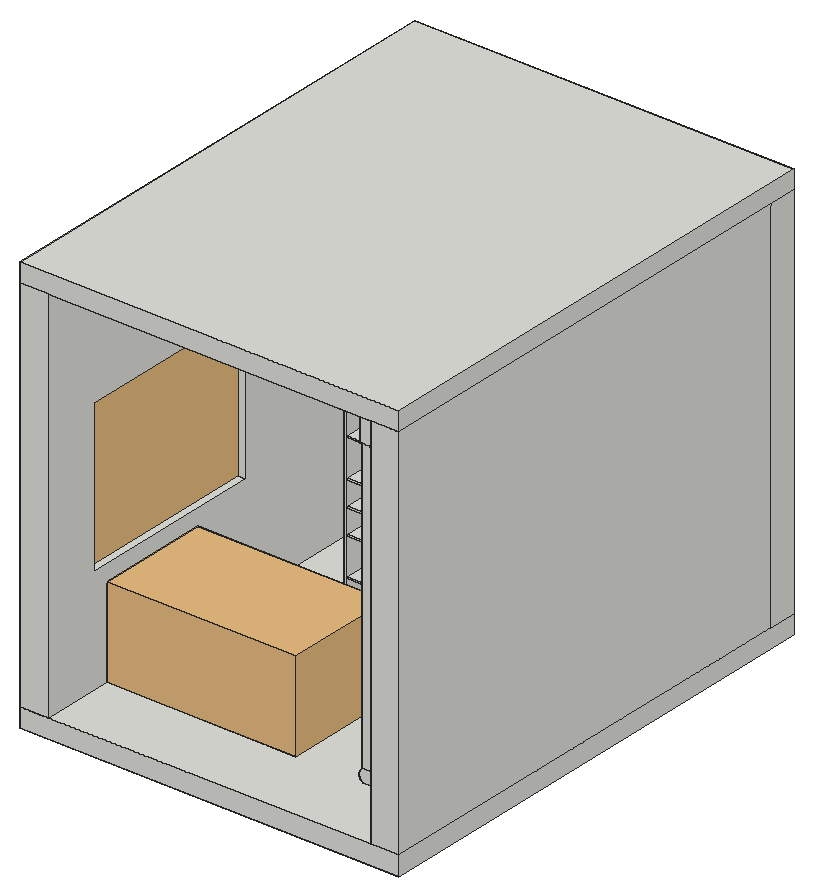
# SketchUp Ruby script. Lengths in inches.
U = 1.inch
M = Sketchup.active_model
def pt(a) = Geom::Point3d.new(a.map { |v| v * U })
def face(e, loops, mat)
  f = e.add_face(loops[0].map { |a| pt(a) })
  loops[1..].each { |l| e.add_face(l.map { |a| pt(a) }).erase! }
  f.material = f.back_material = mat if mat
  f
end
# faces: each face lists its corners as indices into pts; further lists are holes
def faces(e, pts, list, mat = nil) = list.each { |f| face(e, (f[0].is_a?(Array) ? f : [f]).map { |l| l.map { |i| pts[i] } }, mat) }
# xy, xz, yz: faces in a plane at the given z, y or x. An outline is a flat list of corners, or four numbers for a rectangle; further outlines are holes
def ring(l) = l.size == 4 ? [[l[0], l[1]], [l[2], l[1]], [l[2], l[3]], [l[0], l[3]]] : l.each_slice(2).to_a
def flat(e, list, mat, &to3) = list.each { |f| face(e, (f[0].is_a?(Array) ? f : [f]).map { |l| ring(l).map { |u, v| to3.(u, v) } }, mat) }
def xy(e, z, list, mat = nil) = flat(e, list, mat) { |x, y| [x, y, z] }
def xz(e, y, list, mat = nil) = flat(e, list, mat) { |x, z| [x, y, z] }
def yz(e, x, list, mat = nil) = flat(e, list, mat) { |y, z| [x, y, z] }
def lines(e, pts, list) = list.each { |a, b| e.add_line(pt(pts[a]), pt(pts[b])) }
# prism: a flat outline (further loops are holes) pulled along v
def prism(e, loops, v, mat = nil)
  f = face(e, loops, mat); d = Geom::Vector3d.new(v.map { |x| x * U })
  f.pushpull(f.normal.samedirection?(d) ? d.length : -d.length)
end
def box(e, o, s, mat = nil) = prism(e, [[o, [o[0] + s[0], o[1], o[2]], [o[0] + s[0], o[1] + s[1], o[2]], [o[0], o[1] + s[1], o[2]]]], [0, 0, s[2]], mat)
def at(x, y, z, deg = 0) = Geom::Transformation.translation(pt([x, y, z])) * Geom::Transformation.rotation(ORIGIN, Z_AXIS, deg.degrees)
def axes(o, x, y, z) = Geom::Transformation.new([*x, 0, *y, 0, *z, 0, *pt(o).to_a, 1])
def part(name) = M.definitions.add(name)
# library, detail: a bought-in or finely detailed component or shape, given as its bounding box
def library(name, o, s) = part(name).tap { |d| box(d.entities, o, s) }
def detail(e, o, s) = box(e.add_group.entities, o, s)
def put(e, d, t, mat = nil) = e.add_instance(d, t).tap { |i| i.material = mat if mat }
def group(e, t, mat = nil) = e.add_group.tap { |g| g.transformation = t; g.material = mat if mat }.entities
root = M.entities
M.materials.add("[Color C01]").color = [255, 229, 204]
c1 = library("36\" LINEAR DRAIN",[0,0,0],[36,3.67,1.375])
c2 = library("vaso sanitario",[83.83,-83.27,-7.09],[14.69,23.62,31.37])
c3 = library("Health Faucet",[-0.24,4.77,0],[3.42,7.46,21.65])
c4 = library("CUA SO 1",[-70.87,1.66,4.22],[70.87,3.46,66.92])
c5 = library("Casaco",[0,0,0],[25.87,38.71,37.25])
c6 = part("Group\#13")
box(c6.entities,[0,0,0],[9,19,0.5])
c7 = part("Group\#15")
box(c7.entities,[0,0,0],[21,46.71,0.5])
c8 = library("Grupuj\#4",[0,0.09,0],[19.96,5.84,7.875])
c9 = library("Grupuj\#16",[0,0,0],[1.8,5.91,8.5])
c10 = library("Różnica",[0,0,0],[1.2,1.2,6.8])
c11 = part("Grupuj\#13")
xz(c11.entities,0,[[0.78,0.08,0.96,0.1,1.125,0.17,1.27,0.28,1.38,0.43,1.45,0.6,1.48,0.78,1.45,0.96,1.38,1.125,1.27,1.27,1.125,1.38,0.96,1.45,0.78,1.48,0.6,1.45,0.43,1.38,0.28,1.27,0.17,1.125,0.1,0.96,0.08,0.78,0.1,0.6,0.17,0.43,0.28,0.28,0.43,0.17,0.6,0.1]])
xz(c11.entities,1.22,[[0.78,0,0.58,0.03,0.39,0.1,0.23,0.23,0.1,0.39,0.03,0.58,0,0.78,0.03,0.98,0.1,1.17,0.23,1.33,0.39,1.45,0.58,1.53,0.78,1.56,0.98,1.53,1.17,1.45,1.33,1.33,1.45,1.17,1.53,0.98,1.56,0.78,1.53,0.58,1.45,0.39,1.33,0.23,1.17,0.1,0.98,0.03]])
p = [[0.6,0,0.1],[0.43,0,0.17],[0.39,0.08,0.1],[0.58,0.08,0.03],[0.78,0,0.08],[0.78,0.08,0],
  [0.96,0,0.1],[0.98,0.08,0.03],[1.125,0,0.17],[1.17,0.08,0.1],[0.58,1.22,0.03],[0.39,1.22,0.1],
  [0.78,1.22,0],[0.98,1.22,0.03],[1.17,1.22,0.1],[0.28,0,0.28],[0.23,0.08,0.23],[1.27,0,0.28],
  [1.33,0.08,0.23],[0.23,1.22,0.23],[1.33,1.22,0.23],[0.17,0,0.43],[0.1,0.08,0.39],[1.38,0,0.43],
  [1.45,0.08,0.39],[0.1,1.22,0.39],[1.45,1.22,0.39],[0.1,0,0.6],[0.03,0.08,0.58],[1.45,0,0.6],
  [1.53,0.08,0.58],[0.03,1.22,0.58],[1.53,1.22,0.58],[0.08,0,0.78],[0,0.08,0.78],[1.48,0,0.78],
  [1.56,0.08,0.78],[0,1.22,0.78],[1.56,1.22,0.78],[0.1,0,0.96],[0.03,0.08,0.98],[1.45,0,0.96],
  [1.53,0.08,0.98],[0.03,1.22,0.98],[1.53,1.22,0.98],[0.17,0,1.125],[0.1,0.08,1.17],[1.38,0,1.125],
  [1.45,0.08,1.17],[0.1,1.22,1.17],[1.45,1.22,1.17],[0.28,0,1.27],[0.23,0.08,1.33],[1.27,0,1.27],
  [1.33,0.08,1.33],[0.23,1.22,1.33],[1.33,1.22,1.33],[0.43,0,1.38],[0.39,0.08,1.45],[1.125,0,1.38],
  [1.17,0.08,1.45],[0.39,1.22,1.45],[1.17,1.22,1.45],[0.6,0,1.45],[0.58,0.08,1.53],[0.96,0,1.45],
  [0.98,0.08,1.53],[0.78,0,1.48],[0.78,0.08,1.56],[0.58,1.22,1.53],[0.78,1.22,1.56],[0.98,1.22,1.53]]
faces(c11.entities,p,[[0,1,2,3],[4,0,3,5],[6,4,5,7],[8,6,7,9],[10,3,2,11],[12,5,3,10],[13,7,5,12],[14,9,7,13],
  [1,15,16,2],[17,8,9,18],[11,2,16,19],[20,18,9,14],[15,21,22,16],[23,17,18,24],[19,16,22,25],[26,24,18,20],
  [21,27,28,22],[29,23,24,30],[25,22,28,31],[32,30,24,26],[27,33,34,28],[35,29,30,36],[31,28,34,37],[38,36,30,32],
  [33,39,40,34],[41,35,36,42],[37,34,40,43],[44,42,36,38],[39,45,46,40],[47,41,42,48],[43,40,46,49],[50,48,42,44],
  [45,51,52,46],[53,47,48,54],[49,46,52,55],[56,54,48,50],[51,57,58,52],[59,53,54,60],[55,52,58,61],[62,60,54,56],
  [57,63,64,58],[65,59,60,66],[63,67,68,64],[67,65,66,68],[61,58,64,69],[69,64,68,70],[70,68,66,71],[71,66,60,62]])
c12 = part("Grupuj\#14")
xy(c12.entities,0,[[0.24,0,0.18,0.01,0.12,0.03,0.07,0.07,0.03,0.12,0.01,0.18,0,0.24,0.01,0.3,0.03,0.35,0.07,0.4,0.12,0.44,0.18,0.46,0.24,0.47,0.3,0.46,0.35,0.44,0.4,0.4,0.44,0.35,0.46,0.3,0.47,0.24,0.46,0.18,0.44,0.12,0.4,0.07,0.35,0.03,0.3,0.01]])
xy(c12.entities,1.34,[[0.2,0.08,0.28,0.08,0.31,0.1,0.35,0.125,0.37,0.16,0.39,0.2,0.39,0.28,0.37,0.31,0.35,0.35,0.31,0.37,0.28,0.39,0.2,0.39,0.16,0.37,0.125,0.35,0.1,0.31,0.08,0.28,0.08,0.2,0.1,0.16,0.125,0.125,0.16,0.1]])
p = [[0.07,0.07,1.26],[0.07,0.07,0],[0.12,0.03,0],[0.12,0.03,1.26],[0.18,0.01,0],[0.18,0.01,1.26],
  [0.24,0,1.26],[0.24,0,0],[0.3,0.01,0],[0.3,0.01,1.26],[0.35,0.03,0],[0.35,0.03,1.26],
  [0.4,0.07,0],[0.4,0.07,1.26],[0.03,0.12,1.26],[0.03,0.12,0],[0.01,0.18,1.26],[0.01,0.18,0],
  [0.44,0.12,1.26],[0.44,0.12,0],[0.46,0.18,0],[0.46,0.18,1.26],[0.01,0.3,1.26],[0.01,0.3,0],
  [0,0.24,0],[0,0.24,1.26],[0.47,0.24,0],[0.47,0.24,1.26],[0.46,0.3,0],[0.46,0.3,1.26],
  [0.03,0.35,1.26],[0.03,0.35,0],[0.44,0.35,0],[0.44,0.35,1.26],[0.07,0.4,1.26],[0.07,0.4,0],
  [0.18,0.46,1.26],[0.18,0.46,0],[0.12,0.44,0],[0.12,0.44,1.26],[0.35,0.44,1.26],[0.35,0.44,0],
  [0.3,0.46,0],[0.3,0.46,1.26],[0.4,0.4,1.26],[0.4,0.4,0],[0.24,0.47,0],[0.24,0.47,1.26],
  [0.2,0.08,1.34],[0.16,0.1,1.34],[0.125,0.125,1.34],[0.24,0.08,1.34],[0.28,0.08,1.34],[0.35,0.125,1.34],
  [0.31,0.1,1.34],[0.1,0.16,1.34],[0.08,0.2,1.34],[0.37,0.16,1.34],[0.39,0.2,1.34],[0.08,0.24,1.34],
  [0.08,0.28,1.34],[0.39,0.28,1.34],[0.39,0.24,1.34],[0.1,0.31,1.34],[0.125,0.35,1.34],[0.16,0.37,1.34],
  [0.35,0.35,1.34],[0.37,0.31,1.34],[0.31,0.37,1.34],[0.2,0.39,1.34],[0.24,0.39,1.34],[0.28,0.39,1.34]]
faces(c12.entities,p,[[0,1,2,3],[3,2,4,5],[6,7,8,9],[5,4,7,6],[9,8,10,11],[11,10,12,13],[14,15,1,0],[16,17,15,14],
  [18,19,20,21],[13,12,19,18],[22,23,24,25],[25,24,17,16],[21,20,26,27],[27,26,28,29],[30,31,23,22],[29,28,32,33],
  [34,35,31,30],[36,37,38,39],[39,38,35,34],[40,41,42,43],[44,45,41,40],[33,32,45,44],[43,42,46,47],[47,46,37,36],
  [48,49,3,5],[49,50,0,3],[51,48,5,6],[52,51,6,9],[53,54,11,13],[54,52,9,11],[50,55,14,0],[55,56,16,14],
  [57,53,13,18],[58,57,18,21],[59,60,22,25],[56,59,25,16],[61,62,27,29],[62,58,21,27],[63,64,34,30],[60,63,30,22],
  [64,65,39,34],[66,67,33,44],[68,66,44,40],[67,61,29,33],[65,69,36,39],[70,71,43,47],[69,70,47,36],[71,68,40,43]])
c13 = part("Grupuj\#15")
put(c13.entities,c11,at(0,0,0))
put(c13.entities,c12,at(0.54,0.31,1.22))
c14 = part("Grupuj\#10")
xy(c14.entities,0,[[0.47,0.11,0.38,0.125,0.29,0.16,0.22,0.22,0.16,0.29,0.125,0.38,0.11,0.47,0.125,0.57,0.16,0.65,0.22,0.73,0.29,0.78,0.38,0.82,0.47,0.83,0.57,0.82,0.65,0.78,0.73,0.73,0.78,0.65,0.82,0.57,0.83,0.47,0.82,0.38,0.78,0.29,0.73,0.22,0.65,0.16,0.57,0.125]])
xy(c14.entities,1.85,[[0.47,0,0.59,0.02,0.71,0.0625,0.81,0.14,0.88,0.24,0.93,0.35,0.94,0.47,0.93,0.59,0.88,0.71,0.81,0.81,0.71,0.88,0.59,0.93,0.47,0.94,0.35,0.93,0.24,0.88,0.14,0.81,0.0625,0.71,0.02,0.59,0,0.47,0.02,0.35,0.0625,0.24,0.14,0.14,0.24,0.0625,0.35,0.02]])
p = [[0.38,0.125,0],[0.35,0.02,1.85],[0.24,0.0625,1.85],[0.29,0.16,0],[0.47,0.11,0],[0.47,0,1.85],
  [0.57,0.125,0],[0.59,0.02,1.85],[0.65,0.16,0],[0.71,0.0625,1.85],[0.14,0.14,1.85],[0.0625,0.24,1.85],
  [0.16,0.29,0],[0.22,0.22,0],[0.73,0.22,0],[0.81,0.14,1.85],[0.78,0.29,0],[0.88,0.24,1.85],
  [0.02,0.35,1.85],[0.125,0.38,0],[0.82,0.38,0],[0.93,0.35,1.85],[0,0.47,1.85],[0.11,0.47,0],
  [0.83,0.47,0],[0.94,0.47,1.85],[0.02,0.59,1.85],[0.125,0.57,0],[0.82,0.57,0],[0.93,0.59,1.85],
  [0.0625,0.71,1.85],[0.16,0.65,0],[0.78,0.65,0],[0.88,0.71,1.85],[0.22,0.73,0],[0.14,0.81,1.85],
  [0.24,0.88,1.85],[0.29,0.78,0],[0.65,0.78,0],[0.71,0.88,1.85],[0.81,0.81,1.85],[0.73,0.73,0],
  [0.35,0.93,1.85],[0.38,0.82,0],[0.47,0.94,1.85],[0.47,0.83,0],[0.59,0.93,1.85],[0.57,0.82,0]]
faces(c14.entities,p,[[0,1,2,3],[4,5,1,0],[6,7,5,4],[8,9,7,6],[10,11,12,13],[3,2,10,13],[14,15,9,8],[15,14,16,17],
  [11,18,19,12],[17,16,20,21],[18,22,23,19],[21,20,24,25],[22,26,27,23],[24,28,29,25],[27,26,30,31],[28,32,33,29],
  [34,35,36,37],[31,30,35,34],[38,39,40,41],[32,41,40,33],[37,36,42,43],[43,42,44,45],[45,44,46,47],[47,46,39,38]])
c15 = part("Różnica\#5")
xz(c15.entities,0,[[0.778,0,0.979,0.026,1.166,0.104,1.327,0.228,1.451,0.389,1.529,0.576,1.555,0.778,1.529,0.979,1.451,1.166,1.327,1.327,1.166,1.451,0.979,1.529,0.778,1.555,0.576,1.529,0.389,1.451,0.228,1.327,0.104,1.166,0.026,0.979,0,0.778,0.026,0.576,0.104,0.389,0.228,0.228,0.389,0.104,0.576,0.026]])
xz(c15.entities,0.789,[[0.474,0.069,0.469,0.071,0.469,0.126],[1.081,0.069,1.143,0.868,1.143,0.094]])
xz(c15.entities,1.217,[[0.469,0.156,0.428,0.173,0.284,0.284,0.173,0.428,0.103,0.597,0.079,0.778,0.103,0.958,0.173,1.127,0.284,1.271,0.428,1.382,0.469,1.399],[1.143,0.185,1.143,1.37,1.271,1.271,1.382,1.127,1.452,0.958,1.476,0.778,1.452,0.597,1.382,0.428,1.271,0.284]])
yz(c15.entities,0.469,[[0.789,0.071,1.138,0.071,1.217,0.156,1.217,1.399,1.138,1.484,0.913,1.484,0.877,1.014,0.789,0.126]])
yz(c15.entities,1.143,[[0.789,0.094,0.789,0.868,0.848,1.461,1.138,1.461,1.185,1.41,1.217,1.37,1.217,0.185,1.185,0.145,1.138,0.094]])
p = [[0.389,1.138,0.104],[0.469,1.138,0.071],[0.469,0.789,0.071],[0.474,0.789,0.069],[0.449,0.758,0.079],[0.411,0.667,0.095],
  [0.397,0.569,0.101],[0.411,0.471,0.095],[0.449,0.379,0.079],[0.511,0.302,0.054],[0.576,0.254,0.026],[0.576,0,0.026],
  [0.389,0,0.104],[0.59,0.244,0.025],[0.681,0.207,0.013],[0.778,0.195,0],[0.778,0,0],[0.875,0.207,0.013],
  [0.965,0.244,0.025],[0.979,0.254,0.026],[0.979,0,0.026],[1.106,0.758,0.079],[1.081,0.789,0.069],[1.143,0.789,0.094],
  [1.143,1.138,0.094],[1.166,1.138,0.104],[1.166,0,0.104],[1.044,0.302,0.054],[1.106,0.379,0.079],[1.144,0.471,0.095],
  [1.158,0.569,0.101],[1.144,0.667,0.095],[0.656,0.117,1.539],[0.544,0.165,1.515],[0.576,0.151,1.529],[0.778,0.1,1.555],
  [0.899,0.117,1.539],[1.011,0.165,1.515],[0.979,0.151,1.529],[0.449,0.241,1.476],[1.106,0.241,1.476],[0.228,0,0.228],
  [0.228,1.138,0.228],[1.327,1.138,0.228],[1.327,0,0.228],[0.377,0.338,1.442],[0.389,0.322,1.451],[1.178,0.338,1.442],
  [1.166,0.322,1.451],[0.333,0.45,1.408],[1.222,0.45,1.408],[0.318,0.569,1.397],[1.237,0.569,1.397],[0.333,0.688,1.408],
  [1.222,0.688,1.408],[0.377,0.8,1.442],[1.178,0.8,1.442],[0.469,0.789,0.126],[0.469,0.877,1.014],[0.449,0.897,1.476],
  [0.389,0.816,1.451],[1.166,0.816,1.451],[1.143,0.848,1.461],[1.143,0.789,0.868],[0.284,1.217,0.284],[0.428,1.217,0.173],
  [0.469,1.217,0.156],[1.143,1.185,0.145],[1.143,1.217,0.185],[1.271,1.217,0.284],[0.104,0,0.389],[0.104,1.138,0.389],
  [1.451,1.138,0.389],[1.451,0,0.389],[0.173,1.217,0.428],[1.382,1.217,0.428],[0.026,0,0.576],[0.026,1.138,0.576],
  [1.529,1.138,0.576],[1.529,0,0.576],[0.103,1.217,0.597],[1.452,1.217,0.597],[0,0,0.778],[0,1.138,0.778],
  [1.555,1.138,0.778],[1.555,0,0.778],[0.079,1.217,0.778],[1.476,1.217,0.778],[0.026,0,0.979],[0.026,1.138,0.979],
  [1.529,1.138,0.979],[1.529,0,0.979],[0.103,1.217,0.958],[1.452,1.217,0.958],[0.104,0,1.166],[0.104,1.138,1.166],
  [1.451,1.138,1.166],[1.451,0,1.166],[0.469,0.913,1.484],[0.173,1.217,1.127],[1.382,1.217,1.127],[0.284,1.217,1.271],
  [0.228,1.138,1.327],[1.271,1.217,1.271],[1.327,1.138,1.327],[0.228,0,1.327],[1.327,0,1.327],[0.389,0,1.451],
  [0.389,1.138,1.451],[1.166,1.138,1.451],[1.166,0,1.451],[0.428,1.217,1.382],[1.143,1.217,1.37],[1.143,1.185,1.41],
  [0.469,1.138,1.484],[0.469,1.217,1.399],[1.143,1.138,1.461],[0.576,0,1.529],[0.778,0,1.555],[0.979,0,1.529]]
faces(c15.entities,p,[[0,1,2,3,4,5,6,7,8,9,10,11,12],[11,10,13,14,15,16],[16,15,17,18,19,20],[21,22,23,24,25,26,20,19,27,28,29,30,31],[32,14,13,33,34],[35,15,14,32],[36,17,15,35],[37,18,17,36,38],
  [33,13,10,9,39],[40,27,19,18,37],[41,42,0,12],[26,25,43,44],[39,9,8,45,46],[47,28,27,40,48],[45,8,7,49],[50,29,28,47],
  [49,7,6,51],[29,50,52,30],[51,6,5,53],[54,31,30,52],[53,5,4,55],[56,21,31,54],[4,3,57,58,59,60,55],[61,62,63,22,21,56],
  [64,65,0,42],[65,66,1,0],[25,67,68,69,43],[25,24,67],[70,71,42,41],[44,43,72,73],[74,64,42,71],[69,75,72,43],
  [76,77,71,70],[73,72,78,79],[80,74,71,77],[75,81,78,72],[82,83,77,76],[79,78,84,85],[86,80,77,83],[81,87,84,78],
  [88,89,83,82],[85,84,90,91],[92,86,83,89],[87,93,90,84],[94,95,89,88],[91,90,96,97],[59,58,98],[99,92,89,95],
  [93,100,96,90],[101,99,95,102],[100,103,104,96],[105,102,95,94],[97,96,104,106],[107,46,45,49,51,53,55,60,108,102,105],[109,61,56,54,52,50,47,48,110,106,104],[111,101,102,108],
  [103,112,113,109,104],[108,114,115,111],[109,113,116],[117,34,33,39,46,107],[118,35,32,34,117],[119,38,36,35,118],[110,48,40,37,38,119],[59,98,114,108,60],
  [109,116,62,61]])
c16 = part("Różnica\#1")
xz(c16.entities,0,[[0.78,0,0.98,0.03,1.17,0.1,1.33,0.23,1.45,0.39,1.53,0.58,1.56,0.78,1.53,0.98,1.45,1.17,1.33,1.33,1.17,1.45,0.98,1.53,0.78,1.56,0.58,1.53,0.39,1.45,0.23,1.33,0.1,1.17,0.03,0.98,0,0.78,0.03,0.58,0.1,0.39,0.23,0.23,0.39,0.1,0.58,0.03]])
xz(c16.entities,1.72,[[0.78,0,0.58,0.03,0.39,0.1,0.23,0.23,0.1,0.39,0.03,0.58,0,0.78,0.03,0.98,0.1,1.17,0.23,1.33,0.39,1.45,0.58,1.53,0.78,1.56,0.98,1.53,1.17,1.45,1.33,1.33,1.45,1.17,1.53,0.98,1.56,0.78,1.53,0.58,1.45,0.39,1.33,0.23,1.17,0.1,0.98,0.03]])
p = [[0.58,1.72,0.03],[0.58,1.125,0.03],[0.57,1.12,0.03],[0.51,1.04,0.05],[0.47,0.9375,0.07],[0.45,0.83,0.08],
  [0.47,0.73,0.07],[0.51,0.625,0.05],[0.57,0.54,0.03],[0.58,0.54,0.03],[0.58,0,0.03],[0.39,0,0.1],
  [0.39,1.72,0.1],[0.66,0.48,0.02],[0.76,0.4375,0],[0.78,0.43,0],[0.78,0,0],[0.86,0.42,0.01],
  [0.97,0.4375,0.03],[0.98,0.4375,0.03],[0.98,0,0.03],[1.07,0.48,0.0625],[1.15,0.54,0.1],[1.17,0.56,0.1],
  [1.17,0,0.1],[0.66,0.48,1.54],[0.76,0.4375,1.55],[0.78,0.43,1.56],[0.86,0.42,1.54],[0.97,0.4375,1.53],
  [0.98,0.4375,1.53],[1.07,0.48,1.49],[0.51,0.625,1.5],[0.57,0.54,1.53],[0.58,0.54,1.53],[0.57,1.12,1.53],
  [0.51,1.04,1.5],[0.78,1.72,0],[0.78,1.23,0],[0.76,1.23,0],[0.66,1.1875,0.02],[0.66,1.1875,1.54],
  [0.58,1.125,1.53],[1.17,1.72,0.1],[1.17,1.11,0.1],[1.15,1.12,0.1],[1.07,1.1875,0.0625],[0.98,1.22,0.03],
  [0.98,1.72,0.03],[0.76,1.23,1.55],[0.97,1.23,0.03],[0.86,1.24,0.01],[0.86,1.24,1.54],[0.78,1.23,1.56],
  [0.97,1.23,1.53],[1.07,1.1875,1.49],[0.98,1.22,1.53],[0.23,1.72,0.23],[0.23,0,0.23],[1.22,0.625,0.15],
  [1.26,0.73,0.18],[1.27,0.83,0.1875],[1.26,0.9375,0.18],[1.22,1.04,0.15],[1.33,1.72,0.23],[1.33,0,0.23],
  [1.15,0.54,1.46],[1.17,0.56,1.45],[1.22,0.625,1.41],[0.47,0.73,1.48],[1.26,0.73,1.38],[0.45,0.83,1.48],
  [0.47,0.9375,1.48],[1.22,1.04,1.41],[1.26,0.9375,1.38],[1.15,1.12,1.46],[1.17,1.11,1.45],[0.1,1.72,0.39],
  [0.1,0,0.39],[1.45,1.72,0.39],[1.45,0,0.39],[1.27,0.83,1.37],[0.03,1.72,0.58],[0.03,0,0.58],
  [1.53,1.72,0.58],[1.53,0,0.58],[0,1.72,0.78],[0,0,0.78],[1.56,1.72,0.78],[1.56,0,0.78],
  [0.03,1.72,0.98],[0.03,0,0.98],[1.53,1.72,0.98],[1.53,0,0.98],[0.1,1.72,1.17],[0.1,0,1.17],
  [1.45,1.72,1.17],[1.45,0,1.17],[0.23,1.72,1.33],[0.23,0,1.33],[1.33,1.72,1.33],[1.33,0,1.33],
  [0.39,1.72,1.45],[0.39,0,1.45],[1.17,1.72,1.45],[1.17,0,1.45],[0.58,0,1.53],[0.58,1.72,1.53],
  [0.78,0,1.56],[0.98,0,1.53],[0.78,1.72,1.56],[0.98,1.72,1.53]]
faces(c16.entities,p,[[0,1,2,3,4,5,6,7,8,9,10,11,12],[10,9,13,14,15,16],[16,15,17,18,19,20],[20,19,21,22,23,24],[13,25,26,14],[14,26,27,28,17,15],[29,18,17,28],[18,29,30,31,21,19],
  [7,32,33,8],[8,33,34,25,13,9],[2,35,36,3],[37,38,39,40,1,0],[40,41,42,35,2,1],[43,44,45,46,47,48],[39,49,41,40],[48,47,50,51,38,37],
  [51,52,53,49,39,38],[50,54,52,51],[46,55,56,54,50,47],[57,12,11,58],[24,23,59,60,61,62,63,44,43,64,65],[21,31,66,22],[22,66,67,68,59,23],[6,69,32,7],
  [70,60,59,68],[5,71,69,6],[4,72,71,5],[3,36,72,4],[73,63,62,74],[75,45,44,63,73,76],[45,75,55,46],[77,57,58,78],
  [64,79,80,65],[81,61,60,70],[74,62,61,81],[82,77,78,83],[79,84,85,80],[86,82,83,87],[84,88,89,85],[90,86,87,91],
  [88,92,93,89],[94,90,91,95],[92,96,97,93],[98,94,95,99],[96,100,101,97],[102,98,99,103],[104,76,73,74,81,70,68,67,105,101,100],[106,34,33,32,69,71,72,36,35,42,107,102,103],
  [108,27,26,25,34,106],[109,30,29,28,27,108],[105,67,66,31,30,109],[107,42,41,49,53,110],[111,56,55,75,76,104],[110,53,52,54,56,111]])
c17 = part("Grupuj\#8")
xy(c17.entities,0,[[0.39,0.08,0.3125,0.09,0.24,0.12,0.17,0.17,0.12,0.24,0.09,0.3125,0.08,0.39,0.09,0.48,0.12,0.55,0.17,0.62,0.24,0.67,0.3125,0.7,0.39,0.71,0.48,0.7,0.55,0.67,0.62,0.62,0.67,0.55,0.7,0.48,0.71,0.39,0.7,0.3125,0.67,0.24,0.62,0.17,0.55,0.12,0.48,0.09]])
xy(c17.entities,26.57,[[0.39,0.08,0.48,0.09,0.55,0.12,0.62,0.17,0.67,0.24,0.7,0.3125,0.71,0.39,0.7,0.48,0.67,0.55,0.62,0.62,0.55,0.67,0.48,0.7,0.39,0.71,0.3125,0.7,0.24,0.67,0.17,0.62,0.12,0.55,0.09,0.48,0.08,0.39,0.09,0.3125,0.12,0.24,0.17,0.17,0.24,0.12,0.3125,0.09]])
p = [[0.29,0.01,0.08],[0.2,0.05,0.08],[0.24,0.12,0],[0.3125,0.09,0],[0.39,0,0.08],[0.39,0.08,0],
  [0.5,0.01,0.08],[0.48,0.09,0],[0.59,0.05,0.08],[0.55,0.12,0],[0.12,0.12,0.08],[0.17,0.17,0],
  [0.05,0.2,0.08],[0.12,0.24,0],[0.73,0.2,0.08],[0.67,0.12,0.08],[0.62,0.17,0],[0.67,0.24,0],
  [0.01,0.29,0.08],[0.09,0.3125,0],[0.77,0.29,0.08],[0.7,0.3125,0],[0,0.39,0.08],[0.08,0.39,0],
  [0.79,0.39,0.08],[0.71,0.39,0],[0.01,0.5,0.08],[0.09,0.48,0],[0.77,0.5,0.08],[0.7,0.48,0],
  [0.05,0.59,0.08],[0.12,0.55,0],[0.73,0.59,0.08],[0.67,0.55,0],[0.12,0.67,0.08],[0.17,0.62,0],
  [0.2,0.73,0.08],[0.24,0.67,0],[0.59,0.73,0.08],[0.67,0.67,0.08],[0.62,0.62,0],[0.55,0.67,0],
  [0.29,0.77,0.08],[0.3125,0.7,0],[0.39,0.79,0.08],[0.39,0.71,0],[0.5,0.77,0.08],[0.48,0.7,0],
  [0.29,0.01,26.5],[0.2,0.05,26.5],[0.39,0,26.5],[0.5,0.01,26.5],[0.59,0.05,26.5],[0.12,0.12,26.5],
  [0.05,0.2,26.5],[0.67,0.12,26.5],[0.73,0.2,26.5],[0.01,0.29,26.5],[0.77,0.29,26.5],[0,0.39,26.5],
  [0.79,0.39,26.5],[0.01,0.5,26.5],[0.77,0.5,26.5],[0.05,0.59,26.5],[0.73,0.59,26.5],[0.12,0.67,26.5],
  [0.67,0.67,26.5],[0.2,0.73,26.5],[0.29,0.77,26.5],[0.5,0.77,26.5],[0.59,0.73,26.5],[0.39,0.79,26.5],
  [0.3125,0.09,26.57],[0.24,0.12,26.57],[0.39,0.08,26.57],[0.48,0.09,26.57],[0.55,0.12,26.57],[0.17,0.17,26.57],
  [0.12,0.24,26.57],[0.62,0.17,26.57],[0.67,0.24,26.57],[0.09,0.3125,26.57],[0.7,0.3125,26.57],[0.08,0.39,26.57],
  [0.71,0.39,26.57],[0.09,0.48,26.57],[0.7,0.48,26.57],[0.12,0.55,26.57],[0.67,0.55,26.57],[0.17,0.62,26.57],
  [0.24,0.67,26.57],[0.62,0.62,26.57],[0.55,0.67,26.57],[0.3125,0.7,26.57],[0.39,0.71,26.57],[0.48,0.7,26.57]]
faces(c17.entities,p,[[0,1,2,3],[4,0,3,5],[6,4,5,7],[8,6,7,9],[1,10,11,2],[10,12,13,11],[14,15,16,17],[15,8,9,16],
  [12,18,19,13],[20,14,17,21],[18,22,23,19],[24,20,21,25],[22,26,27,23],[28,24,25,29],[26,30,31,27],[32,28,29,33],
  [30,34,35,31],[34,36,37,35],[38,39,40,41],[39,32,33,40],[36,42,43,37],[42,44,45,43],[44,46,47,45],[46,38,41,47],
  [48,49,1,0],[50,48,0,4],[51,50,4,6],[52,51,6,8],[49,53,10,1],[53,54,12,10],[55,52,8,15],[56,55,15,14],
  [54,57,18,12],[58,56,14,20],[57,59,22,18],[60,58,20,24],[59,61,26,22],[62,60,24,28],[61,63,30,26],[64,62,28,32],
  [63,65,34,30],[66,64,32,39],[65,67,36,34],[67,68,42,36],[69,70,38,46],[70,66,39,38],[68,71,44,42],[71,69,46,44],
  [72,73,49,48],[74,72,48,50],[75,74,50,51],[76,75,51,52],[77,78,54,53],[73,77,53,49],[79,76,52,55],[80,79,55,56],
  [78,81,57,54],[82,80,56,58],[81,83,59,57],[84,82,58,60],[83,85,61,59],[86,84,60,62],[85,87,63,61],[88,86,62,64],
  [89,90,67,65],[87,89,65,63],[91,88,64,66],[92,91,66,70],[90,93,68,67],[93,94,71,68],[94,95,69,71],[95,92,70,69]])
c18 = part("Grupuj\#17")
put(c18.entities,c17,at(0.99,0.42,0))
c19 = library("Group\#31",[-0.37,0,0],[47.8,48,28.35])
xz(root,99.82,[[85.46,34.23,85.54,34.23,85.55,35.76,85.47,35.76],[85.47,35.76,85.55,35.76,85.56,36.8125,85.48,36.8125]],"[Color C01]")
xz(root,100.41,[[85.48,32.07,85.48,34.23,85.55,34.23,85.5625,32.07]],"[Color C01]")
yz(root,85.22,[[100.09,32.08,100.08,34.23,100.16,34.23,100.16,32.08],[100.08,34.23,100.16,35.76]],"[Color C01]")
p = [[84.65,99.21,21.94],[84.6,99.27,21.94],[85.1,99.75,22.49],[85.16,99.6875,22.49],[84.69,99.15,21.96],[85.2,99.625,22.5],
  [84.54,99.32,21.96],[85.04,99.79,22.5],[84.75,99.04,22.05],[84.73,99.09,22],[85.22,99.55,22.53],[85.22,99.48,22.5625],
  [84.76,98.99,22.11],[85.21,99.42,22.6],[84.49,99.36,22],[84.97,99.8125,22.53],[84.43,99.39,22.05],[84.9,99.82,22.56],
  [84.75,98.96,22.1875],[85.18,99.36,22.65],[84.39,99.4,22.12],[84.36,99.39,22.19],[84.78,99.78,22.65],[84.83,99.8125,22.6],
  [84.73,98.94,22.26],[85.13,99.32,22.7],[84.34,99.37,22.27],[84.73,99.74,22.69],[84.7,98.94,22.33],[85.07,99.29,22.74],
  [84.65,98.95,22.4],[85.01,99.28,22.78],[84.33,99.34,22.34],[84.34,99.29,22.41],[84.68,99.62,22.78],[84.7,99.68,22.74],
  [84.6,98.97,22.45],[84.9375,99.29,22.82],[84.36,99.24,22.46],[84.6875,99.55,22.81],[84.55,99.01,22.49],[84.87,99.3125,22.84],
  [84.49,99.0625,22.51],[84.8,99.36,22.85],[84.4375,99.12,22.51],[84.75,99.41,22.85],[84.39,99.18,22.5],[84.71,99.48,22.84],
  [85.46,99.8,23.42],[85.46,99.73,23.43],[85.41,99.95,23.4],[85.45,99.88,23.41],[85.29,100.04,23.4],[85.35,100,23.4],
  [85.14,100.07,23.43],[85.22,100.0625,23.41],[85.4,99.59,23.47],[85.35,99.54,23.49],[85.44,99.66,23.45],[84.94,99.96,23.48],
  [85,100.01,23.46],[85.07,100.05,23.44],[85.28,99.5,23.51],[85.21,99.49,23.52],[84.89,99.82,23.52],[84.91,99.9,23.5],
  [85.06,99.51,23.55],[84.99,99.55,23.55],[85.13,99.49,23.54],[84.94,99.61,23.55],[84.9,99.67,23.54],[84.88,99.75,23.53],
  [85.57,99.8,24.92],[85.53,99.74,24.93],[85.6,99.88,24.91],[85.6,99.95,24.91],[85.58,100.03,24.9],[85.49,100.15,24.9],
  [85.54,100.1,24.9],[85.13,100.16,24.92],[85.2,100.2,24.92],[85.27,100.22,24.91],[85.35,100.21,24.9],[85.42,100.19,24.9],
  [85.1875,99.65,24.96],[85.12,99.69,24.96],[85.34,99.63,24.95],[85.26,99.63,24.95],[85.41,99.65,24.94],[85.48,99.69,24.9375],
  [85.07,99.75,24.96],[85.03,99.82,24.96],[85.01,99.89,24.95],[85.01,99.97,24.94],[85.03,100.04,24.9375],[85.07,100.11,24.93],
  [85.51,99.76,27.23],[85.43,99.74,27.23],[85.35,99.74,27.23],[85.57,99.8,27.22],[85.67,99.92,27.21],[85.63,99.85,27.22],
  [85.69,99.99,27.21],[85.11,100,27.23],[85.11,100.08,27.23],[85.69,100.07,27.21],[85.13,100.16,27.22],[85.17,100.22,27.22],
  [85.64,100.21,27.2],[85.67,100.14,27.21],[85.22,100.27,27.22],[85.58,100.27,27.2],[85.29,100.3125,27.21],[85.37,100.33,27.21],
  [85.44,100.33,27.21],[85.52,100.31,27.2],[85.28,99.77,27.23],[85.16,99.86,27.23],[85.125,99.93,27.23],[85.21,99.81,27.23],
  [85.41,99.81,29.56],[85.34,99.83,29.56],[85.57,99.82,29.55],[85.49,99.8,29.55],[85.27,99.87,29.56],[85.22,99.92,29.56],
  [85.63,99.86,29.55],[85.69,99.91,29.55],[85.18,99.99,29.56],[85.17,100.07,29.56],[85.73,99.98,29.54],[85.75,100.05,29.54],
  [85.17,100.14,29.55],[85.75,100.13,29.54],[85.1875,100.22,29.55],[85.7,100.27,29.54],[85.73,100.2,29.54],[85.23,100.28,29.55],
  [85.28,100.34,29.55],[85.64,100.33,29.54],[85.35,100.37,29.55],[85.43,100.39,29.54],[85.5,100.39,29.54],[85.58,100.37,29.54],
  [85.69,99.88,32.07],[85.625,99.84,32.08],[85.75,99.93,32.07],[85.79,100,32.07],[85.81,100.07,32.07],[85.79,100.22,32.07],
  [85.81,100.15,32.07],[85.75,100.29,32.07],[85.34,100.36,32.07],[85.29,100.3,32.08],[85.41,100.39,32.07],[85.7,100.35,32.07],
  [85.64,100.39,32.07],[85.5625,100.41,32.07],[85.48,100.41,32.07],[85.47,99.83,32.08],[85.4,99.85,32.08],[85.33,99.89,32.08],
  [85.55,99.82,32.08],[85.28,99.94,32.08],[85.24,100.01,32.08],[85.22,100.09,32.08],[85.22,100.16,32.08],[85.25,100.24,32.08],
  [85.39,99.84,34.23],[85.32,99.88,34.23],[85.46,99.82,34.23],[85.62,99.84,34.23],[85.54,99.82,34.23],[85.68,99.875,34.23],
  [85.27,99.9375,34.23],[85.23,100.01,34.23],[85.74,99.93,34.23],[85.78,99.99,34.23],[85.22,100.08,34.23],[85.8,100.07,34.23],
  [85.8,100.15,34.23],[85.78,100.22,34.23],[85.24,100.23,34.23],[85.28,100.3,34.23],[85.22,100.16,34.23],[85.75,100.29,34.23],
  [85.33,100.35,34.23],[85.63,100.38,34.23],[85.69,100.34,34.23],[85.4,100.39,34.23],[85.48,100.41,34.23],[85.55,100.41,34.23],
  [85.4,99.84,35.76],[85.33,99.88,35.76],[85.47,99.82,35.76],[85.41,99.84,36.8125],[85.62,99.84,35.76],[85.55,99.82,35.76],
  [85.6875,99.87,35.76],[85.28,99.9375,35.76],[85.24,100,35.76],[85.74,99.93,35.75],[85.78,99.99,35.75],[85.22,100.08,35.76],
  [85.81,100.07,35.75],[85.79,100.22,35.75],[85.81,100.14,35.75],[85.24,100.23,35.76],[85.28,100.3,35.76],[85.22,100.16,35.76],
  [85.75,100.29,35.75],[85.34,100.35,35.76],[85.41,100.39,35.76],[85.7,100.34,35.75],[85.63,100.38,35.76],[85.48,100.4,35.76],
  [85.56,100.4,35.76],[85.57,100.4,36.81],[85.34,99.88,36.8125],[85.48,99.82,36.8125],[85.63,99.84,36.8125],[85.56,99.82,36.8125],
  [85.7,99.875,36.81],[85.29,99.9375,36.8125],[85.25,100.01,36.8125],[85.8,99.99,36.81],[85.76,99.93,36.81],[85.23,100.08,36.8125],
  [85.82,100.07,36.81],[85.23,100.16,36.8125],[85.8,100.22,36.81],[85.82,100.14,36.81],[85.26,100.23,36.8125],[85.3,100.3,36.8125],
  [85.76,100.29,36.81],[85.35,100.35,36.8125],[85.42,100.39,36.8125],[85.71,100.34,36.81],[85.64,100.38,36.81],[85.49,100.41,36.8125],
  [572.46,900.37,0],[572.46,900.37,-0.28]]
faces(root,p,[[0,1,2,3],[4,0,3,5],[1,6,7,2],[8,9,10,11],[12,8,11,13],[9,4,5,10],[6,14,15,7],[14,16,17,15],
  [18,12,13,19],[20,21,22,23],[16,20,23,17],[24,18,19,25],[21,26,27,22],[28,24,25,29],[30,28,29,31],[32,33,34,35],
  [26,32,35,27],[36,30,31,37],[33,38,39,34],[40,36,37,41],[42,40,41,43],[44,42,43,45],[46,44,45,47],[38,46,47,39],
  [11,10,48,49],[5,3,50,51],[10,5,51,48],[2,7,52,53],[3,2,53,50],[15,17,54,55],[7,15,55,52],[25,19,56,57],
  [13,11,49,58],[19,13,58,56],[22,27,59,60],[23,22,60,61],[17,23,61,54],[31,29,62,63],[29,25,57,62],[35,34,64,65],
  [27,35,65,59],[43,41,66,67],[37,31,63,68],[41,37,68,66],[47,45,69,70],[39,47,70,71],[34,39,71,64],[45,43,67,69],
  [56,58,72,73],[58,49,74,72],[49,48,75,74],[48,51,76,75],[50,53,77,78],[51,50,78,76],[61,60,79,80],[54,61,80,81],
  [52,55,82,83],[53,52,83,77],[55,54,81,82],[67,66,84,85],[68,63,86,87],[66,68,87,84],[63,62,88,86],[57,56,73,89],
  [62,57,89,88],[69,67,85,90],[70,69,90,91],[71,70,91,92],[64,71,92,93],[65,64,93,94],[59,65,94,95],[60,59,95,79],
  [86,88,96,97],[87,86,97,98],[88,89,99,96],[73,72,100,101],[89,73,101,99],[72,74,102,100],[93,92,103,104],[74,75,105,102],
  [94,93,104,106],[95,94,106,107],[76,78,108,109],[75,76,109,105],[79,95,107,110],[78,77,111,108],[80,79,110,112],[81,80,112,113],
  [82,81,113,114],[83,82,114,115],[77,83,115,111],[84,87,98,116],[91,90,117,118],[85,84,116,119],[90,85,119,117],[92,91,118,103],
  [116,98,120,121],[97,96,122,123],[98,97,123,120],[119,116,121,124],[117,119,124,125],[96,99,126,122],[99,101,127,126],[118,117,125,128],
  [103,118,128,129],[101,100,130,127],[100,102,131,130],[104,103,129,132],[102,105,133,131],[106,104,132,134],[109,108,135,136],[105,109,136,133],
  [107,106,134,137],[110,107,137,138],[108,111,139,135],[112,110,138,140],[113,112,140,141],[114,113,141,142],[115,114,142,143],[111,115,143,139],
  [144,145,122,126],[146,144,126,127],[130,147,146,127],[131,148,147,130],[136,149,150,133],[133,150,148,131],[135,151,149,136],[152,138,137,153],
  [154,140,138,152],[135,139,155,151],[155,139,143,156],[157,142,141,158],[158,141,140,154],[156,143,142,157],[159,160,121,120],[160,161,124,121],
  [162,159,120,123],[145,162,123,122],[128,125,163,164],[124,161,163,125],[129,128,164,165],[134,132,166,167],[132,129,165,166],[137,134,167,153],
  [160,168,169,161],[159,170,168,160],[145,171,172,162],[162,172,170,159],[144,173,171,145],[164,163,174,175],[161,169,174,163],[146,176,173,144],
  [147,177,176,146],[165,164,175,178],[148,179,177,147],[150,180,179,148],[149,181,180,150],[153,167,182,183],[167,166,184,182],[151,185,181,149],
  [152,153,183,186],[155,156,187,188],[151,155,188,185],[154,152,186,189],[158,154,189,190],[156,157,191,187],[192,193,169,168],[170,194,195],
  [192,170,195],[168,170,192],[196,197,172,171],[198,196,171,173],[175,174,199,200],[169,193,199,174],[201,198,173,176],[177,202,201,176],
  [178,175,200,203],[179,204,202,177],[181,205,206,180],[180,206,204,179],[183,182,207,208],[182,184,209,207],[185,210,205,181],[211,186,183,208],
  [212,189,186,211],[213,188,187,214],[185,188,213,210],[215,190,189,212],[216,191,190,215],[187,217,214],[216,217,187],[191,216,187],
  [195,218,193,192],[219,195,194],[220,221,197,196],[222,220,196,198],[199,223,224,200],[193,218,223,199],[202,225,226,201],[226,222,198,201],
  [200,224,227,203],[204,228,225,202],[209,203,227,229],[206,205,230,231],[206,231,228,204],[208,207,232,233],[207,209,229,232],[205,210,234,230],
  [235,211,208,233],[236,212,211,235],[237,213,214,238],[210,213,237,234],[239,215,212,236],[217,216,215,239],[238,214,217],[238,217,239,236,235,233,232,229,227,224,223,218,195,219,221,220,222,226,225,228,231,230,234,237]],"[Color C01]")
lines(root,p,[[240,241]])
put(root,c1,at(53,142.33,8.625))
put(root,c2,at(27.73,31.63,17.09,90))
put(root,c3,at(106.05,128.63,15.95))
put(root,c4,axes([7.54,78,36.32],[0,0.84667,0],[-0.7,0,0],[0,0,0.71718]))
put(root,c5,axes([56.8,92.69,57.66],[0,-0.85,0],[0.85,0,0],[0,0,1.054]))
g1 = group(root,at(0,0,0))
box(g1,[0,0,0],[120,156,6])
g2 = group(root,at(0,36,6))
xy(g2,0,[[0,-36,0,120,120,120,120,111,9,111,9,-36]])
xy(g2,33.35,[[0,-18,9,42]])
xy(g2,81.35,[[0,-18,9,42]])
xy(g2,120,[[0,-36,9,-36,9,111,120,111,120,120,0,120]])
xz(g2,-36,[[0,0,9,120]])
xz(g2,-18,[[0,33.35,9,81.35]])
xz(g2,42,[[0,33.35,9,81.35]])
xz(g2,111,[[9,0,120,120]])
xz(g2,120,[[0,0,120,120]])
yz(g2,0,[[[-36,0,120,120],[-18,33.35,42,81.35]]])
yz(g2,9,[[[-36,0,111,120],[-18,33.35,42,81.35]]])
yz(g2,120,[[111,0,120,120]])
g3 = group(root,at(111,0,6))
box(g3,[0,0,0],[9,147,120])
g4 = group(root,at(0,0,126))
box(g4,[0,0,0],[120,156,6])
g5 = group(root,at(45,93,6))
xy(g5,0,[[0,0,0,54,6,54,6,6,66,6,66,0]])
xy(g5,6,[[0,6,6,36]])
xy(g5,90,[[0,6,6,36]])
xy(g5,108,[[0,0,66,0,66,6,6,6,6,54,0,54]])
xz(g5,0,[[0,0,66,108]])
xz(g5,6,[[6,0,6,6,0,6,0,90,6,90,6,108,66,108,66,0]])
xz(g5,36,[[0,6,6,90]])
xz(g5,54,[[0,0,6,108]])
yz(g5,0,[[[0,0,54,108],[6,6,36,90]]])
yz(g5,6,[[6,0,54,0,54,108,6,108,6,90,36,90,36,6,6,6]])
yz(g5,66,[[0,0,6,108]])
g6 = group(root,at(45,23,6))
xy(g6,0,[[45,0,45,49,0,49,0,70,66,70,66,0]])
xy(g6,4,[[45,0,66,0,66,70,0,70,0,49,45,49]])
xz(g6,0,[[45,0,66,0,66,4,45,4,44.69,3.75,44.43,3.46,44.22,3.13,44.0625,2.77,43.97,2.39,43.9375,2,43.97,1.61,44.0625,1.23,44.22,0.87,44.43,0.54,44.69,0.25]])
xz(g6,49,[[0,0,-0.31,0.25,-0.57,0.54,-0.78,0.87,-0.9375,1.23,-1.03,1.61,-1.0625,2,-1.03,2.39,-0.9375,2.77,-0.78,3.13,-0.57,3.46,-0.31,3.75,0,4]])
xz(g6,70,[[0,0,66,4]])
yz(g6,0,[[49,0,70,4]])
yz(g6,66,[[0,0,70,4]])
p = [[45,0,0],[44.69,0,0.25],[44.69,48.69,0.25],[45,49,0],[-0.31,48.69,0.25],[0,49,0],
  [-0.31,49,0.25],[44.43,0,0.54],[44.43,48.43,0.54],[-0.57,48.43,0.54],[-0.57,49,0.54],[44.22,0,0.87],
  [44.22,48.22,0.87],[-0.78,48.22,0.87],[-0.78,49,0.87],[44.0625,0,1.23],[44.0625,48.0625,1.23],[-0.9375,48.0625,1.23],
  [-0.9375,49,1.23],[43.97,0,1.61],[43.97,47.97,1.61],[-1.03,47.97,1.61],[-1.03,49,1.61],[43.9375,0,2],
  [43.9375,47.9375,2],[-1.0625,47.9375,2],[-1.0625,49,2],[43.97,0,2.39],[43.97,47.97,2.39],[-1.03,47.97,2.39],
  [-1.03,49,2.39],[44.0625,0,2.77],[44.0625,48.0625,2.77],[-0.9375,48.0625,2.77],[-0.9375,49,2.77],[44.22,0,3.13],
  [44.22,48.22,3.13],[-0.78,48.22,3.13],[-0.78,49,3.13],[44.43,0,3.46],[44.43,48.43,3.46],[-0.57,48.43,3.46],
  [-0.57,49,3.46],[44.69,0,3.75],[44.69,48.69,3.75],[-0.31,48.69,3.75],[-0.31,49,3.75],[45,0,4],
  [45,49,4],[0,49,4]]
faces(g6,p,[[0,1,2,3],[3,2,4,5],[5,4,6],[1,7,8,2],[2,8,9,4],[4,9,10,6],[7,11,12,8],[8,12,13,9],
  [9,13,14,10],[11,15,16,12],[12,16,17,13],[13,17,18,14],[15,19,20,16],[16,20,21,17],[17,21,22,18],[19,23,24,20],
  [20,24,25,21],[21,25,26,22],[23,27,28,24],[24,28,29,25],[25,29,30,26],[27,31,32,28],[28,32,33,29],[29,33,34,30],
  [31,35,36,32],[32,36,37,33],[33,37,38,34],[35,39,40,36],[37,41,42,38],[36,40,41,37],[39,43,44,40],[41,45,46,42],
  [40,44,45,41],[43,47,48,44],[45,49,46],[44,48,49,45]])
g7 = group(root,at(45,23,102))
xy(g7,0,[[44,0,44,48,0,48,0,70,66,70,66,0]])
xy(g7,1,[[44,1,65,47],[1,48,43,69]])
xy(g7,11,[[44,1,65,47],[1,48,43,69]])
xy(g7,12,[[44,0,66,0,66,70,0,70,0,48,44,48]])
xz(g7,0,[[44,0,66,12]])
xz(g7,1,[[44,1,65,11]])
xz(g7,47,[[44,1,65,11]])
xz(g7,48,[[[0,0,44,12],[1,1,43,11]]])
xz(g7,69,[[1,1,43,11]])
xz(g7,70,[[0,0,66,12]])
yz(g7,0,[[48,0,70,12]])
yz(g7,1,[[48,1,69,11]])
yz(g7,43,[[48,1,69,11]])
yz(g7,44,[[[0,0,48,12],[1,1,47,11]]])
yz(g7,65,[[1,1,47,11]])
yz(g7,66,[[0,0,70,12]])
g8 = group(root,at(9,23,6))
xy(g8,0,[[0,0,60,36]])
put(root,c6,at(46,71.71,19))
put(root,c6,at(46,71.71,27))
put(root,c6,at(46,71.71,39))
put(root,c6,at(46,71.71,47))
put(root,c6,at(46,71.71,55))
put(root,c6,at(46,71.71,67))
put(root,c6,at(46,71.71,78.17))
put(root,c6,at(46,71.71,89.33))
g9 = group(root,at(56,71.71,55.75))
box(g9,[0,0,0],[32.71,19,0.5])
g10 = group(root,at(45,23,10))
xy(g10,0,[[44.71,0,44.71,48.71,0,48.71,0,70,66,70,66,0]])
xy(g10,1,[[44.71,1,65.71,47.71],[1,48.71,10,69.71],[11,48.71,43.71,68.71]])
xy(g10,91,[[44.71,1,65.71,47.71],[1,48.71,10,69.71],[11,48.71,43.71,68.71]])
xy(g10,92,[[44.71,0,66,0,66,70,0,70,0,48.71,44.71,48.71]])
xz(g10,0,[[44.71,0,66,92]])
xz(g10,1,[[44.71,1,65.71,91]])
xz(g10,47.71,[[44.71,1,65.71,91]])
xz(g10,48.71,[[[0,0,44.71,92],[11,1,43.71,91],[1,1,10,91]]])
xz(g10,68.71,[[11,1,43.71,91]])
xz(g10,69.71,[[1,1,10,91]])
xz(g10,70,[[0,0,66,92]])
yz(g10,0,[[48.71,0,70,92]])
yz(g10,1,[[48.71,1,69.71,91]])
yz(g10,10,[[48.71,1,69.71,91]])
yz(g10,11,[[48.71,1,68.71,91]])
yz(g10,43.71,[[48.71,1,68.71,91]])
yz(g10,44.71,[[[0,0,48.71,92],[1,1,47.71,91]]])
yz(g10,65.71,[[1,1,47.71,91]])
yz(g10,66,[[0,0,70,92]])
put(root,c7,at(89.71,24,20.5))
put(root,c7,at(89.71,24,30))
put(root,c7,at(89.71,24,39.5))
put(root,c7,at(89.71,24,49))
put(root,c7,at(89.71,24,61.5))
g11 = group(root,at(51,99,6))
xy(g11,0,[[0,0,60,48]])
xy(g11,2.5,[[2,43.33,38,47]])
xy(g11,4,[[[0,0,60,48],[2,43.33,38,47]]])
xz(g11,0,[[0,0,60,4]])
xz(g11,43.33,[[2,2.5,38,4]])
xz(g11,47,[[2,2.5,38,4]])
xz(g11,48,[[0,0,60,4]])
yz(g11,0,[[0,0,48,4]])
yz(g11,2,[[43.33,2.5,47,4]])
yz(g11,38,[[43.33,2.5,47,4]])
yz(g11,60,[[0,0,48,4]])
g12 = group(root,at(53.96,143.65,8))
xy(g12,0,[[0,0,19.125,2.5]])
g13 = group(root,at(53,142,8.5))
xy(g13,0,[[0,0,36,4]])
put(root,c8,axes([70.97,99,94],[0,1,0],[0,0,1],[1,0,0]),"[Color C01]")
put(root,c9,at(77.77,99,46,90),"[Color C01]")
put(root,c10,axes([84.53,99.67,51.86],[0,0.84121,-0.2717],[-0.884,0,0],[0,0.31246,0.96739]),"[Color C01]")
put(root,c13,at(87.51,99.16,50.1875,90),"[Color C01]")
put(root,c14,axes([84.47,99.17,50.125],[0,0.95159,-0.30736],[-1,0,0],[0,0.30736,0.95159]),"[Color C01]")
put(root,c15,axes([84.57,98.96,50.45],[0,0.95159,-0.30736],[-1,0,0],[0,0.30736,0.95159]),"[Color C01]")
put(root,c16,axes([86.26,99.19,50.22],[0,0.96,0],[-0.96,0,0],[0,0,0.96]),"[Color C01]")
put(root,c18,at(86.28,98.64,36.73,90),"[Color C01]")
put(root,c19,axes([69,23.28,6],[0,0.75315,0],[-1.25,0,0],[0,0,1]))
